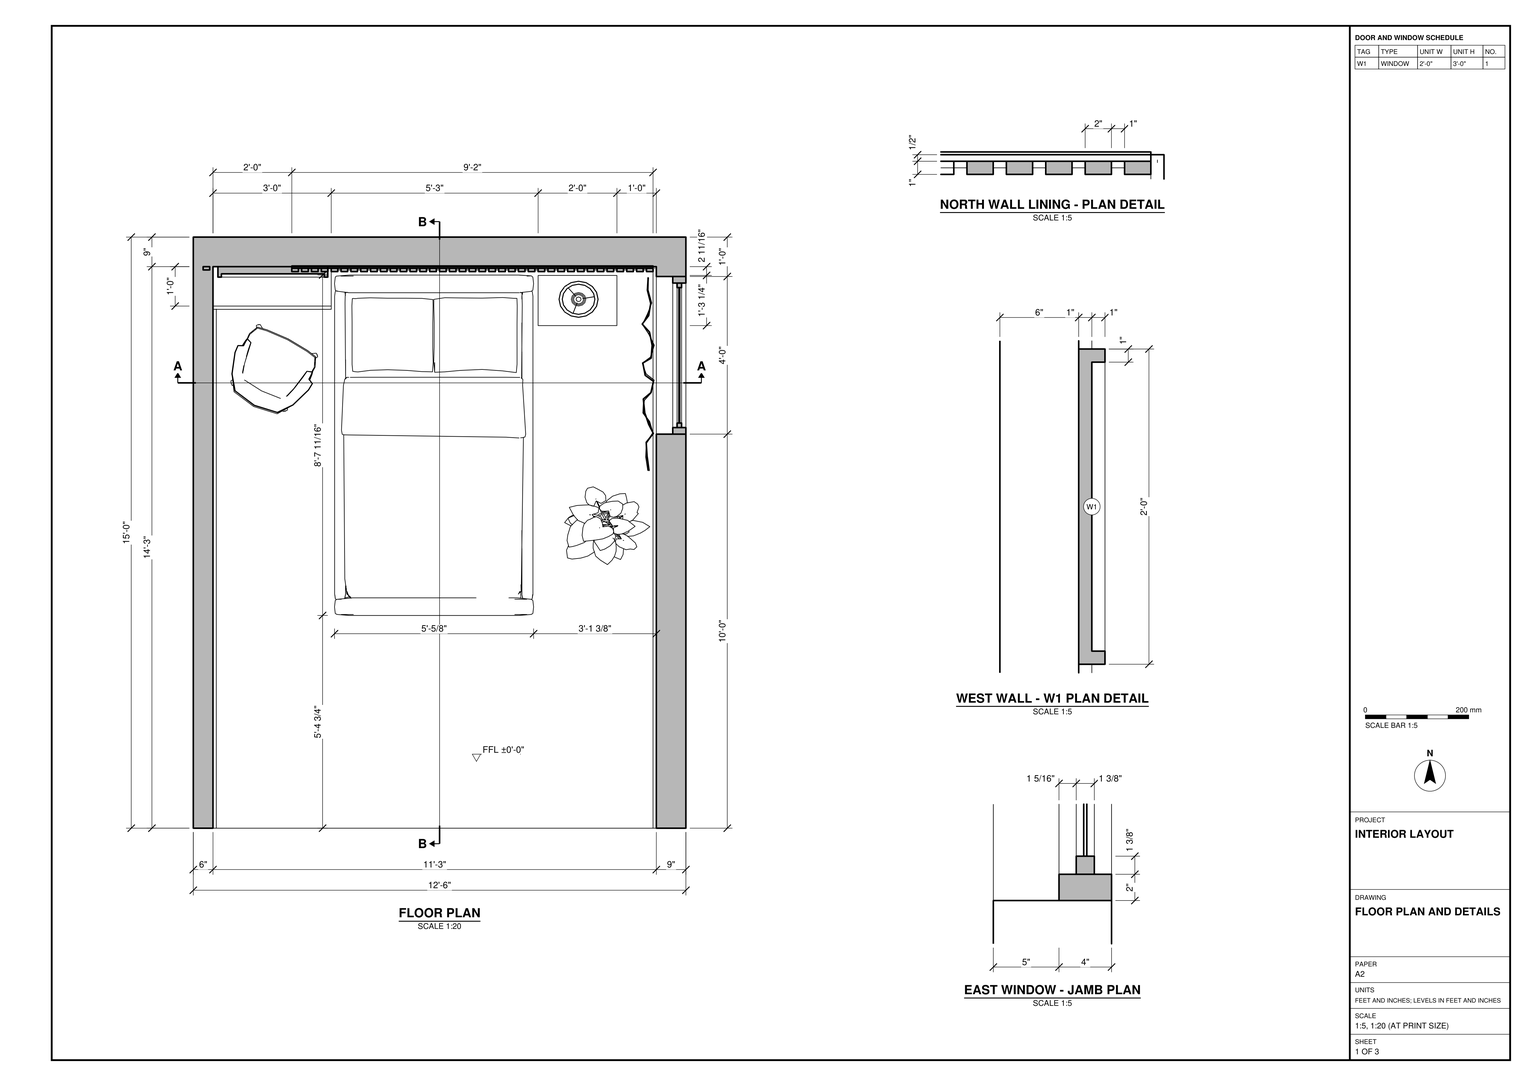
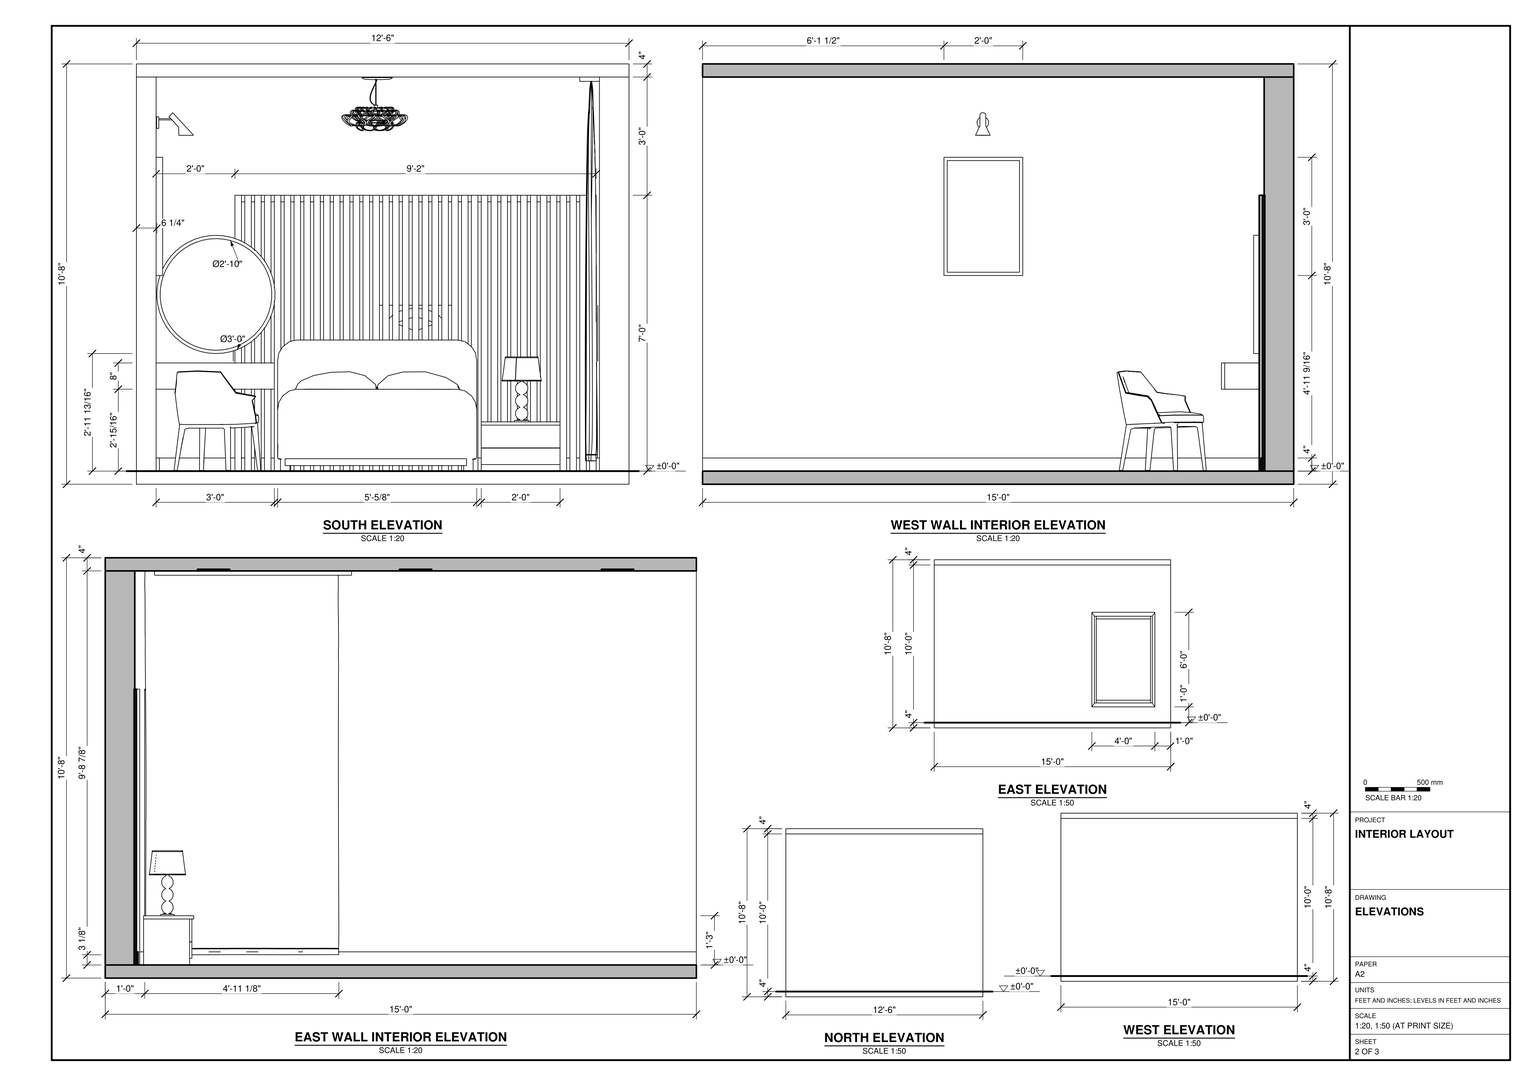
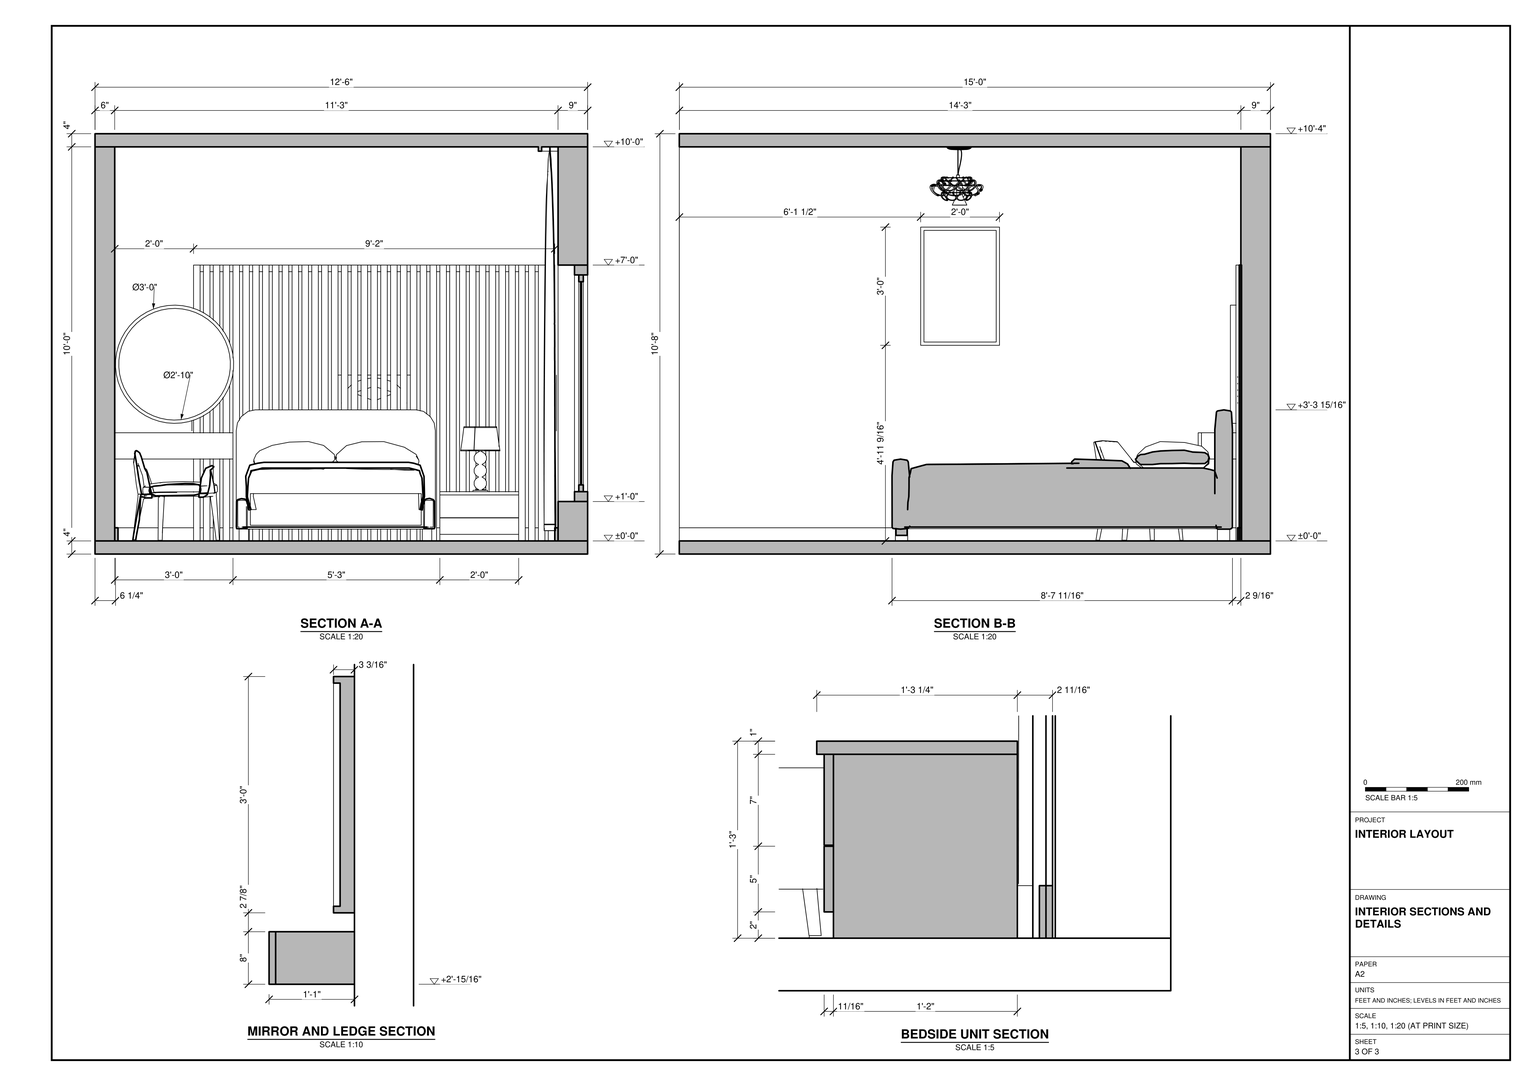
Build the bedroom in SketchUp from task_files/diagram_01.pdf. Work in feet and inches. The room shell measures 12'-6" across by 15'-0" deep and 10'-8" high overall. Set the finished floor at ±0'-0". Model the floor and ceiling slabs, each 4" thick, with a clear height of 10'-0" between them. Leave the south side open as drawn. Make the west wall 6" thick and the north and east walls 9" thick. Use the plan, elevations and jamb detail to place the east window, and include the smaller framed unit shown on the inside of the west wall.

Run the vertical slatted lining across the north wall as dimensioned. Set the bed with its head against the lining and its foot toward the open side. To the left of the bed, model the wall-mounted ledge with the round mirror above and the chair in front. To the right, model the low bedside unit using its section detail. Place the bedside lamp, curtains, plant, ceiling light and wall light where shown. Decor and loose items may be any suitable library components.

Keep the walls and slabs and each furniture or joinery piece in separate groups or components, and use components for repeated parts. Save one SketchUp model as output_files/furnished_bedroom_with_a_slatted_headboard_wall.skp.

# SketchUp Ruby script. Lengths in inches.
U = 1.inch
M = Sketchup.active_model
def pt(a) = Geom::Point3d.new(a.map { |v| v * U })
def face(e, loops, mat)
  f = e.add_face(loops[0].map { |a| pt(a) })
  loops[1..].each { |l| e.add_face(l.map { |a| pt(a) }).erase! }
  f.material = f.back_material = mat if mat
  f
end
# faces: each face lists its corners as indices into pts; further lists are holes
def faces(e, pts, list, mat = nil) = list.each { |f| face(e, (f[0].is_a?(Array) ? f : [f]).map { |l| l.map { |i| pts[i] } }, mat) }
# xy, xz, yz: faces in a plane at the given z, y or x. An outline is a flat list of corners, or four numbers for a rectangle; further outlines are holes
def ring(l) = l.size == 4 ? [[l[0], l[1]], [l[2], l[1]], [l[2], l[3]], [l[0], l[3]]] : l.each_slice(2).to_a
def flat(e, list, mat, &to3) = list.each { |f| face(e, (f[0].is_a?(Array) ? f : [f]).map { |l| ring(l).map { |u, v| to3.(u, v) } }, mat) }
def xy(e, z, list, mat = nil) = flat(e, list, mat) { |x, y| [x, y, z] }
def xz(e, y, list, mat = nil) = flat(e, list, mat) { |x, z| [x, y, z] }
def yz(e, x, list, mat = nil) = flat(e, list, mat) { |y, z| [x, y, z] }
def lines(e, pts, list) = list.each { |a, b| e.add_line(pt(pts[a]), pt(pts[b])) }
# prism: a flat outline (further loops are holes) pulled along v
def prism(e, loops, v, mat = nil)
  f = face(e, loops, mat); d = Geom::Vector3d.new(v.map { |x| x * U })
  f.pushpull(f.normal.samedirection?(d) ? d.length : -d.length)
end
def box(e, o, s, mat = nil) = prism(e, [[o, [o[0] + s[0], o[1], o[2]], [o[0] + s[0], o[1] + s[1], o[2]], [o[0], o[1] + s[1], o[2]]]], [0, 0, s[2]], mat)
def at(x, y, z, deg = 0) = Geom::Transformation.translation(pt([x, y, z])) * Geom::Transformation.rotation(ORIGIN, Z_AXIS, deg.degrees)
def axes(o, x, y, z) = Geom::Transformation.new([*x, 0, *y, 0, *z, 0, *pt(o).to_a, 1])
def part(name) = M.definitions.add(name)
# library, detail: a bought-in or finely detailed component or shape, given as its bounding box
def library(name, o, s) = part(name).tap { |d| box(d.entities, o, s) }
def detail(e, o, s) = box(e.add_group.entities, o, s)
def put(e, d, t, mat = nil) = e.add_instance(d, t).tap { |i| i.material = mat if mat }
def group(e, t, mat = nil) = e.add_group.tap { |g| g.transformation = t; g.material = mat if mat }.entities
root = M.entities
M.materials.add("0215 AP 9421 FABRIC PINK").color = [153, 66, 100]
M.materials.add("0401 AP 9656 Gulmarg Winters-N").color = [195, 225, 234]
M.materials.add("CTS Window Glass").color = [170, 210, 225]
M.materials["CTS Window Glass"].alpha = 0.45
M.materials.add("Emissive\#1").color = [255, 196, 127]
M.materials.add("[Wood Cherry Original]").color = [152, 86, 42]
c1 = part("Headboard wall slat")
box(c1.entities,[0,-4,0],[2,84,1],"[Wood Cherry Original]")
c2 = library("Light Wall 003",[-2.22,-12.37,-3.88],[4.44,12.37,6.91])
c3 = library("Chair 027",[-12.79,-10.9,0.01],[25.58,23.14,30.54])
c4 = library("Eva Bed",[-34.4,-44.85,0.04],[68.9,90.3,39.91])
c5 = library("Lamp Table 114-10",[-7.7,-7.7,0],[15.4,15.4,24.72])
c6 = library("Indoor Plant 001",[-24.46,-30.5625,0],[48.74,57.4,53.14])
c7 = library("Light",[127.07,-9.39,-4.83],[16.23,16.19,39.83])
c8 = library("Curtains 005",[1.83,-1.86,0.24],[37.77,3.72,116.83])
c9 = part("Group64\#2")
prism(c9.entities,[[[143.75,-49.45,88.01],[143.75,-51.45,86.01],[143.75,-51.45,134.01],[143.75,-49.45,132.01]]],[4,0,0])
c10 = part("Group65\#2")
prism(c10.entities,[[[143.75,-3.45,86.01],[143.75,-5.45,88.01],[143.75,-5.45,132.01],[143.75,-3.45,134.01]]],[4,0,0])
c11 = part("Group66\#2")
prism(c11.entities,[[[143.75,-49.45,132.01],[143.75,-51.45,134.01],[143.75,-3.45,134.01],[143.75,-5.45,132.01]]],[4,0,0])
c12 = part("Group67\#2")
prism(c12.entities,[[[143.75,-51.45,86.01],[143.75,-49.45,88.01],[143.75,-5.45,88.01],[143.75,-3.45,86.01]]],[4,0,0])
c13 = part("Group70\#2")
box(c13.entities,[145.0625,-49.45,88.01],[1.375,1.38,44])
c14 = part("Group71\#2")
box(c14.entities,[145.0625,-6.83,88.01],[1.375,1.38,44])
c15 = part("Group72\#2")
box(c15.entities,[145.0625,-48.07,130.64],[1.375,41.24,1.37])
c16 = part("Group73\#2")
box(c16.entities,[145.0625,-48.07,88.01],[1.375,41.24,1.38])
c17 = part("Group69\#2")
put(c17.entities,c13,at(0,0,0))
put(c17.entities,c14,at(0,0,0))
put(c17.entities,c15,at(0,0,0))
put(c17.entities,c16,at(0,0,0))
c18 = part("Group74\#2")
box(c18.entities,[145.63,-48.07,89.39],[0.24,41.24,41.25],"CTS Window Glass")
c19 = part("Group68\#2")
put(c19.entities,c17,at(0,0,0))
put(c19.entities,c18,at(0,0,0))
c20 = part("CTS_Window_Frame\#1")
put(c20.entities,c9,at(0,0,0))
put(c20.entities,c10,at(0,0,0))
put(c20.entities,c11,at(0,0,0))
put(c20.entities,c12,at(0,0,0))
put(c20.entities,c19,at(0,0,0))
c21 = library("Group\#6",[-0.5,-0.5,0],[111,1,84])
c22 = part("Recessed light pair")
xy(c22.entities,-0.5,[[5.97,1,7.27,1.16,8.47,1.66,9.51,2.44,10.32,3.47,10.82,4.68,11,5.97,10.84,7.27,10.34,8.47,9.56,9.51,8.53,10.32,7.32,10.82,6.03,11,4.73,10.84,3.53,10.34,2.49,9.56,1.68,8.53,1.18,7.32,1,6.03,1.16,4.73,1.66,3.53,2.44,2.49,3.47,1.68,4.68,1.18],[5.97,73,7.27,73.16,8.47,73.66,9.51,74.44,10.32,75.47,10.82,76.68,11,77.97,10.84,79.27,10.34,80.47,9.56,81.51,8.53,82.32,7.32,82.82,6.03,83,4.73,82.84,3.53,82.34,2.49,81.56,1.68,80.53,1.18,79.32,1,78.03,1.16,76.73,1.66,75.53,2.44,74.49,3.47,73.68,4.68,73.18]],"Emissive\#1")
xy(c22.entities,0,[[[5.96,0,7.52,0.2,8.97,0.79,10.22,1.73,11.18,2.97,11.79,4.41,12,5.96,11.8,7.52,11.21,8.97,10.27,10.22,9.03,11.18,7.59,11.79,6.04,12,4.48,11.8,3.03,11.21,1.78,10.27,0.82,9.03,0.21,7.59,0,6.04,0.2,4.48,0.79,3.03,1.73,1.78,2.97,0.82,4.41,0.21],[5.97,1,4.68,1.18,3.47,1.68,2.44,2.49,1.66,3.53,1.16,4.73,1,6.03,1.18,7.32,1.68,8.53,2.49,9.56,3.53,10.34,4.73,10.84,6.03,11,7.32,10.82,8.53,10.32,9.56,9.51,10.34,8.47,10.84,7.27,11,5.97,10.82,4.68,10.32,3.47,9.51,2.44,8.47,1.66,7.27,1.16]],[[5.96,72,7.52,72.2,8.97,72.79,10.22,73.73,11.18,74.97,11.79,76.41,12,77.96,11.8,79.52,11.21,80.97,10.27,82.22,9.03,83.18,7.59,83.79,6.04,84,4.48,83.8,3.03,83.21,1.78,82.27,0.82,81.03,0.21,79.59,0,78.04,0.2,76.48,0.79,75.03,1.73,73.78,2.97,72.82,4.41,72.21],[5.97,73,4.68,73.18,3.47,73.68,2.44,74.49,1.66,75.53,1.16,76.73,1,78.03,1.18,79.32,1.68,80.53,2.49,81.56,3.53,82.34,4.73,82.84,6.03,83,7.32,82.82,8.53,82.32,9.56,81.51,10.34,80.47,10.84,79.27,11,77.97,10.82,76.68,10.32,75.47,9.51,74.44,8.47,73.66,7.27,73.16]]])
p = [[4.68,1.18,0],[5.97,1,0],[5.97,1,-0.5],[4.68,1.18,-0.5],[7.27,1.16,0],[7.27,1.16,-0.5],
  [3.47,1.68,0],[3.47,1.68,-0.5],[8.47,1.66,0],[8.47,1.66,-0.5],[2.44,2.49,0],[2.44,2.49,-0.5],
  [9.51,2.44,0],[9.51,2.44,-0.5],[10.32,3.47,0],[10.32,3.47,-0.5],[1.66,3.53,0],[1.66,3.53,-0.5],
  [1.16,4.73,0],[1.16,4.73,-0.5],[10.82,4.68,0],[10.82,4.68,-0.5],[1,6.03,0],[1,6.03,-0.5],
  [11,5.97,0],[11,5.97,-0.5],[1.18,7.32,0],[1.18,7.32,-0.5],[10.84,7.27,0],[10.84,7.27,-0.5],
  [1.68,8.53,0],[1.68,8.53,-0.5],[10.34,8.47,0],[10.34,8.47,-0.5],[2.49,9.56,0],[2.49,9.56,-0.5],
  [9.56,9.51,0],[9.56,9.51,-0.5],[8.53,10.32,0],[8.53,10.32,-0.5],[3.53,10.34,0],[3.53,10.34,-0.5],
  [4.73,10.84,0],[4.73,10.84,-0.5],[7.32,10.82,0],[7.32,10.82,-0.5],[6.03,11,0],[6.03,11,-0.5],
  [4.68,73.18,0],[5.97,73,0],[5.97,73,-0.5],[4.68,73.18,-0.5],[7.27,73.16,0],[7.27,73.16,-0.5],
  [3.47,73.68,0],[3.47,73.68,-0.5],[8.47,73.66,0],[8.47,73.66,-0.5],[2.44,74.49,0],[2.44,74.49,-0.5],
  [9.51,74.44,0],[9.51,74.44,-0.5],[10.32,75.47,0],[10.32,75.47,-0.5],[1.66,75.53,0],[1.66,75.53,-0.5],
  [1.16,76.73,0],[1.16,76.73,-0.5],[10.82,76.68,0],[10.82,76.68,-0.5],[1,78.03,0],[1,78.03,-0.5],
  [11,77.97,0],[11,77.97,-0.5],[1.18,79.32,0],[1.18,79.32,-0.5],[10.84,79.27,0],[10.84,79.27,-0.5],
  [1.68,80.53,0],[1.68,80.53,-0.5],[10.34,80.47,0],[10.34,80.47,-0.5],[2.49,81.56,0],[2.49,81.56,-0.5],
  [9.56,81.51,0],[9.56,81.51,-0.5],[8.53,82.32,0],[8.53,82.32,-0.5],[3.53,82.34,0],[3.53,82.34,-0.5],
  [4.73,82.84,0],[4.73,82.84,-0.5],[7.32,82.82,0],[7.32,82.82,-0.5],[6.03,83,0],[6.03,83,-0.5]]
faces(c22.entities,p,[[0,1,2,3],[1,4,5,2],[6,0,3,7],[4,8,9,5],[10,6,7,11],[8,12,13,9],[12,14,15,13],[16,10,11,17],
  [18,16,17,19],[14,20,21,15],[22,18,19,23],[20,24,25,21],[26,22,23,27],[24,28,29,25],[30,26,27,31],[28,32,33,29],
  [34,30,31,35],[32,36,37,33],[36,38,39,37],[40,34,35,41],[42,40,41,43],[38,44,45,39],[46,42,43,47],[44,46,47,45],
  [48,49,50,51],[49,52,53,50],[54,48,51,55],[52,56,57,53],[58,54,55,59],[56,60,61,57],[60,62,63,61],[64,58,59,65],
  [66,64,65,67],[62,68,69,63],[70,66,67,71],[68,72,73,69],[74,70,71,75],[72,76,77,73],[78,74,75,79],[76,80,81,77],
  [82,78,79,83],[80,84,85,81],[84,86,87,85],[88,82,83,89],[90,88,89,91],[86,92,93,87],[94,90,91,95],[92,94,95,93]],"Emissive\#1")
put(root,c1,axes([3,171,4],[1,0,0],[0,0,1],[0,-1,0]))
put(root,c2,axes([6.14,85.34,106.12],[0,-1,0],[-0.91,0,0],[0,0,1]))
put(root,c3,axes([23.97,139.31,-0.01],[0.89021,-0.45554,0],[-0.45554,-0.89021,0],[0,0,1]))
put(root,c4,axes([73.27,116.26,-0.04],[0.88,0,0],[0,1.148,0],[0,0,1]))
put(root,c5,axes([117.32,161.07,15],[0.77921,0,0],[0,0.72,0],[0,0,0.8]))
put(root,c6,axes([126.09,92.88,0],[0.5325,0,0],[0,0.4125,0],[0,0,0.75]))
put(root,c7,axes([-94.8125,85.71,105.63],[1.2381,0,0],[0,1,0],[0,0,0.4107]))
put(root,c8,axes([138.53,105.99,2.86],[0,1.56501,0],[1,0,0],[0,0,1.00056]))
put(root,c20,axes([2.25,171.45,-117.02],[1,0,0],[0,1,0],[0,0,1.5]))
put(root,c1,axes([123,170.5,4],[1,0,0],[0,0,1],[0,-1,0]),"[Wood Cherry Original]")
put(root,c1,axes([108,170.5,4],[1,0,0],[0,0,1],[0,-1,0]),"[Wood Cherry Original]")
put(root,c1,axes([120,170.5,4],[1,0,0],[0,0,1],[0,-1,0]),"[Wood Cherry Original]")
put(root,c1,axes([117,170.5,4],[1,0,0],[0,0,1],[0,-1,0]),"[Wood Cherry Original]")
put(root,c1,axes([126,170.5,4],[1,0,0],[0,0,1],[0,-1,0]),"[Wood Cherry Original]")
put(root,c1,axes([135,170.5,4],[1,0,0],[0,0,1],[0,-1,0]),"[Wood Cherry Original]")
put(root,c1,axes([129,170.5,4],[1,0,0],[0,0,1],[0,-1,0]),"[Wood Cherry Original]")
put(root,c1,axes([114,170.5,4],[1,0,0],[0,0,1],[0,-1,0]),"[Wood Cherry Original]")
put(root,c1,axes([93,170.5,4],[1,0,0],[0,0,1],[0,-1,0]),"[Wood Cherry Original]")
put(root,c1,axes([111,170.5,4],[1,0,0],[0,0,1],[0,-1,0]),"[Wood Cherry Original]")
put(root,c1,axes([132,170.5,4],[1,0,0],[0,0,1],[0,-1,0]),"[Wood Cherry Original]")
put(root,c1,axes([87,170.5,4],[1,0,0],[0,0,1],[0,-1,0]),"[Wood Cherry Original]")
put(root,c1,axes([48,170.5,4],[1,0,0],[0,0,1],[0,-1,0]),"[Wood Cherry Original]")
put(root,c1,axes([75,170.5,4],[1,0,0],[0,0,1],[0,-1,0]),"[Wood Cherry Original]")
put(root,c1,axes([81,170.5,4],[1,0,0],[0,0,1],[0,-1,0]),"[Wood Cherry Original]")
put(root,c1,axes([69,170.5,4],[1,0,0],[0,0,1],[0,-1,0]),"[Wood Cherry Original]")
put(root,c1,axes([63,170.5,4],[1,0,0],[0,0,1],[0,-1,0]),"[Wood Cherry Original]")
put(root,c1,axes([90,170.5,4],[1,0,0],[0,0,1],[0,-1,0]),"[Wood Cherry Original]")
put(root,c1,axes([57,170.5,4],[1,0,0],[0,0,1],[0,-1,0]),"[Wood Cherry Original]")
put(root,c1,axes([60,170.5,4],[1,0,0],[0,0,1],[0,-1,0]),"[Wood Cherry Original]")
put(root,c1,axes([84,170.5,4],[1,0,0],[0,0,1],[0,-1,0]),"[Wood Cherry Original]")
put(root,c1,axes([51,170.5,4],[1,0,0],[0,0,1],[0,-1,0]),"[Wood Cherry Original]")
put(root,c1,axes([78,170.5,4],[1,0,0],[0,0,1],[0,-1,0]),"[Wood Cherry Original]")
put(root,c1,axes([66,170.5,4],[1,0,0],[0,0,1],[0,-1,0]),"[Wood Cherry Original]")
put(root,c1,axes([72,170.5,4],[1,0,0],[0,0,1],[0,-1,0]),"[Wood Cherry Original]")
put(root,c1,axes([54,170.5,4],[1,0,0],[0,0,1],[0,-1,0]),"[Wood Cherry Original]")
put(root,c1,axes([39,170.5,4],[1,0,0],[0,0,1],[0,-1,0]),"[Wood Cherry Original]")
put(root,c1,axes([36,170.5,4],[1,0,0],[0,0,1],[0,-1,0]),"[Wood Cherry Original]")
put(root,c1,axes([30,170.5,4],[1,0,0],[0,0,1],[0,-1,0]),"[Wood Cherry Original]")
put(root,c1,axes([33,170.5,4],[1,0,0],[0,0,1],[0,-1,0]),"[Wood Cherry Original]")
put(root,c1,axes([42,170.5,4],[1,0,0],[0,0,1],[0,-1,0]),"[Wood Cherry Original]")
put(root,c1,axes([138,170.5,4],[1,0,0],[0,0,1],[0,-1,0]),"[Wood Cherry Original]")
put(root,c1,axes([45,170.5,4],[1,0,0],[0,0,1],[0,-1,0]),"[Wood Cherry Original]")
put(root,c1,axes([99,170.5,4],[1,0,0],[0,0,1],[0,-1,0]),"[Wood Cherry Original]")
put(root,c1,axes([96,170.5,4],[1,0,0],[0,0,1],[0,-1,0]),"[Wood Cherry Original]")
put(root,c1,axes([102,170.5,4],[1,0,0],[0,0,1],[0,-1,0]),"[Wood Cherry Original]")
put(root,c1,axes([105,170.5,4],[1,0,0],[0,0,1],[0,-1,0]),"[Wood Cherry Original]")
g1 = group(root,at(6,180,0,-90))
prism(g1,[[[0,-6,0],[0,0,0],[0,144,0],[0,144,-4],[0,-6,-4]]],[180,0,0])
g2 = group(root,at(6,0,0))
prism(g2,[[[135,171,0],[135,0,0],[134,0,0],[134,170,0],[1,170,0],[1,0,0],[0,0,0],[0,171,0]]],[0,0,4])
g3 = group(root,at(0,0,0))
xy(g3,0,[[0,0,0,180,150,180,150,0,141,0,141,171,6,171,6,0]])
xy(g3,12,[[141,120,150,168]])
xy(g3,84,[[141,120,150,168]])
xy(g3,120,[[0,0,6,0,6,171,141,171,141,0,150,0,150,180,0,180]])
xz(g3,0,[[0,0,6,120],[141,0,150,120]])
xz(g3,120,[[141,12,150,84]])
xz(g3,168,[[141,12,150,84]])
xz(g3,171,[[6,0,141,120]],"0401 AP 9656 Gulmarg Winters-N")
xz(g3,180,[[0,0,150,120]])
yz(g3,0,[[0,0,180,120]])
yz(g3,6,[[0,0,171,120]],"0401 AP 9656 Gulmarg Winters-N")
yz(g3,141,[[[0,0,171,120],[120,12,168,84]]],"0401 AP 9656 Gulmarg Winters-N")
yz(g3,150,[[[0,0,180,120],[120,12,168,84]]])
g4 = group(g3,at(6,73.5,59.5625))
xy(g4,0,[[0,0,2,24]])
xy(g4,1,[[1,1,2,23]])
xy(g4,35,[[1,1,2,23]])
xy(g4,36,[[0,0,2,24]])
xz(g4,0,[[0,0,2,36]])
xz(g4,1,[[1,1,2,35]])
xz(g4,23,[[1,1,2,35]])
xz(g4,24,[[0,0,2,36]])
yz(g4,0,[[0,0,24,36]])
yz(g4,1,[[1,1,23,35]])
yz(g4,2,[[[0,0,24,36],[1,1,23,35]]])
put(root,c21,at(30,170.5,0))
g5 = group(root,at(6.25,167.8125,35.8),"0215 AP 9421 FABRIC PINK")
xz(g5,0,[[[17.79,0,20.05,0.12,22.27,0.52,24.43,1.2,26.49,2.14,28.41,3.33,30.16,4.75,31.73,6.38,33.07,8.2,34.18,10.17,35.04,12.26,35.62,14.45,35.93,16.69,35.95,18.95,35.69,21.19,35.15,23.39,34.34,25.5,33.27,27.49,31.96,29.33,30.43,30.99,28.7,32.45,26.81,33.68,24.77,34.67,22.63,35.39,20.41,35.83,18.16,36,15.9,35.88,13.68,35.48,11.52,34.8,9.47,33.86,7.54,32.67,5.79,31.25,4.22,29.61,2.875,27.8,1.77,25.83,0.91,23.74,0.33,21.55,0.02,19.3125,0,17.05,0.26,14.81,0.8,12.61,1.61,10.5,2.68,8.51,3.99,6.67,5.52,5,7.25,3.55,9.14,2.31,11.18,1.33,13.32,0.61,15.54,0.16],[17.8,1,15.67,1.16,13.58,1.58,11.56,2.26,9.63,3.1875,7.84,4.35,6.21,5.73,4.77,7.3,3.53,9.04,2.52,10.92,1.75,12.91,1.24,14.98,1,17.11,1.02,19.24,1.31,21.36,1.86,23.42,2.67,25.39,3.72,27.25,4.99,28.97,6.47,30.51,8.125,31.85,9.9375,32.98,11.88,33.87,13.92,34.51,16.02,34.89,18.15,35,20.28,34.84,22.37,34.42,24.39,33.74,26.32,32.8125,28.11,31.65,29.74,30.27,31.18,28.7,32.42,26.96,33.43,25.08,34.2,23.09,34.71,21.01,34.95,18.89,34.93,16.76,34.64,14.64,34.09,12.58,33.28,10.6,32.23,8.74,30.96,7.03,29.49,5.49,27.83,4.14,26.01,3.02,24.07,2.13,22.03,1.49,19.93,1.11]]])
xz(g5,1,[[17.8,1,19.93,1.11,22.03,1.49,24.07,2.13,26.01,3.02,27.83,4.14,29.49,5.49,30.96,7.03,32.23,8.74,33.28,10.6,34.09,12.58,34.64,14.64,34.93,16.76,34.95,18.89,34.71,21.01,34.2,23.09,33.43,25.08,32.42,26.96,31.18,28.7,29.74,30.27,28.11,31.65,26.32,32.8125,24.39,33.74,22.37,34.42,20.28,34.84,18.15,35,16.02,34.89,13.92,34.51,11.88,33.87,9.9375,32.98,8.125,31.85,6.47,30.51,4.99,28.97,3.72,27.25,2.67,25.39,1.86,23.42,1.31,21.36,1.02,19.24,1,17.11,1.24,14.98,1.75,12.91,2.52,10.92,3.53,9.04,4.77,7.3,6.21,5.73,7.84,4.35,9.63,3.1875,11.56,2.26,13.58,1.58,15.67,1.16]])
xz(g5,3.1875,[[17.79,0,15.54,0.16,13.32,0.61,11.18,1.33,9.14,2.31,7.25,3.55,5.52,5,3.99,6.67,2.68,8.51,1.61,10.5,0.8,12.61,0.26,14.81,0,17.05,0.02,19.3125,0.33,21.55,0.91,23.74,1.77,25.83,2.875,27.8,4.22,29.61,5.79,31.25,7.54,32.67,9.47,33.86,11.52,34.8,13.68,35.48,15.9,35.88,18.16,36,20.41,35.83,22.63,35.39,24.77,34.67,26.81,33.68,28.7,32.45,30.43,30.99,31.96,29.33,33.27,27.49,34.34,25.5,35.15,23.39,35.69,21.19,35.95,18.95,35.93,16.69,35.62,14.45,35.04,12.26,34.18,10.17,33.07,8.2,31.73,6.38,30.16,4.75,28.41,3.33,26.49,2.14,24.43,1.2,22.27,0.52,20.05,0.12]])
p = [[15.54,3.1875,0.16],[17.79,3.1875,0],[17.79,0,0],[15.54,0,0.16],[20.05,3.1875,0.12],[20.05,0,0.12],
  [22.27,3.1875,0.52],[22.27,0,0.52],[13.32,3.1875,0.61],[13.32,0,0.61],[24.43,3.1875,1.2],[24.43,0,1.2],
  [11.18,3.1875,1.33],[11.18,0,1.33],[15.67,0,1.16],[17.8,0,1],[17.8,1,1],[15.67,1,1.16],
  [19.93,0,1.11],[19.93,1,1.11],[22.03,0,1.49],[22.03,1,1.49],[13.58,0,1.58],[13.58,1,1.58],
  [26.49,3.1875,2.14],[26.49,0,2.14],[9.14,3.1875,2.31],[9.14,0,2.31],[24.07,0,2.13],[24.07,1,2.13],
  [11.56,0,2.26],[11.56,1,2.26],[26.01,0,3.02],[26.01,1,3.02],[28.41,3.1875,3.33],[28.41,0,3.33],
  [7.25,3.1875,3.55],[7.25,0,3.55],[9.63,0,3.1875],[9.63,1,3.1875],[27.83,0,4.14],[27.83,1,4.14],
  [7.84,0,4.35],[7.84,1,4.35],[30.16,3.1875,4.75],[30.16,0,4.75],[5.52,3.1875,5],[5.52,0,5],
  [29.49,0,5.49],[29.49,1,5.49],[6.21,0,5.73],[6.21,1,5.73],[31.73,3.1875,6.38],[31.73,0,6.38],
  [3.99,3.1875,6.67],[3.99,0,6.67],[30.96,0,7.03],[30.96,1,7.03],[4.77,0,7.3],[4.77,1,7.3],
  [33.07,3.1875,8.2],[33.07,0,8.2],[2.68,3.1875,8.51],[2.68,0,8.51],[32.23,0,8.74],[32.23,1,8.74],
  [3.53,0,9.04],[3.53,1,9.04],[34.18,3.1875,10.17],[34.18,0,10.17],[1.61,3.1875,10.5],[1.61,0,10.5],
  [33.28,0,10.6],[33.28,1,10.6],[2.52,0,10.92],[2.52,1,10.92],[35.04,3.1875,12.26],[35.04,0,12.26],
  [0.8,3.1875,12.61],[0.8,0,12.61],[34.09,0,12.58],[34.09,1,12.58],[1.75,0,12.91],[1.75,1,12.91],
  [35.62,3.1875,14.45],[35.62,0,14.45],[0.26,3.1875,14.81],[0.26,0,14.81],[34.64,0,14.64],[34.64,1,14.64],
  [1.24,0,14.98],[1.24,1,14.98],[35.93,3.1875,16.69],[35.93,0,16.69],[34.93,0,16.76],[34.93,1,16.76],
  [0,3.1875,17.05],[0,0,17.05],[1,0,17.11],[1,1,17.11],[35.95,3.1875,18.95],[35.95,0,18.95],
  [34.95,0,18.89],[34.95,1,18.89],[0.02,3.1875,19.3125],[0.02,0,19.3125],[1.02,0,19.24],[1.02,1,19.24],
  [34.71,0,21.01],[34.71,1,21.01],[35.69,3.1875,21.19],[35.69,0,21.19],[1.31,0,21.36],[1.31,1,21.36],
  [0.33,3.1875,21.55],[0.33,0,21.55],[34.2,0,23.09],[34.2,1,23.09],[35.15,3.1875,23.39],[35.15,0,23.39],
  [1.86,0,23.42],[1.86,1,23.42],[0.91,3.1875,23.74],[0.91,0,23.74],[33.43,0,25.08],[33.43,1,25.08],
  [2.67,0,25.39],[2.67,1,25.39],[34.34,3.1875,25.5],[34.34,0,25.5],[1.77,3.1875,25.83],[1.77,0,25.83],
  [32.42,0,26.96],[32.42,1,26.96],[3.72,0,27.25],[3.72,1,27.25],[33.27,3.1875,27.49],[33.27,0,27.49],
  [2.875,3.1875,27.8],[2.875,0,27.8],[31.18,0,28.7],[31.18,1,28.7],[4.99,0,28.97],[4.99,1,28.97],
  [31.96,3.1875,29.33],[31.96,0,29.33],[4.22,3.1875,29.61],[4.22,0,29.61],[29.74,0,30.27],[29.74,1,30.27],
  [6.47,0,30.51],[6.47,1,30.51],[30.43,3.1875,30.99],[30.43,0,30.99],[5.79,3.1875,31.25],[5.79,0,31.25],
  [28.11,0,31.65],[28.11,1,31.65],[8.125,0,31.85],[8.125,1,31.85],[28.7,3.1875,32.45],[28.7,0,32.45],
  [7.54,3.1875,32.67],[7.54,0,32.67],[26.32,0,32.8125],[26.32,1,32.8125],[9.9375,0,32.98],[9.9375,1,32.98],
  [26.81,3.1875,33.68],[26.81,0,33.68],[9.47,3.1875,33.86],[9.47,0,33.86],[24.39,0,33.74],[24.39,1,33.74],
  [11.88,0,33.87],[11.88,1,33.87],[22.37,0,34.42],[22.37,1,34.42],[24.77,3.1875,34.67],[24.77,0,34.67],
  [11.52,3.1875,34.8],[11.52,0,34.8],[13.92,0,34.51],[13.92,1,34.51],[20.28,0,34.84],[20.28,1,34.84],
  [16.02,0,34.89],[16.02,1,34.89],[22.63,3.1875,35.39],[22.63,0,35.39],[13.68,3.1875,35.48],[13.68,0,35.48],
  [18.15,0,35],[18.15,1,35],[20.41,3.1875,35.83],[20.41,0,35.83],[15.9,3.1875,35.88],[15.9,0,35.88],
  [18.16,3.1875,36],[18.16,0,36]]
faces(g5,p,[[0,1,2,3],[1,4,5,2],[4,6,7,5],[8,0,3,9],[6,10,11,7],[12,8,9,13],[14,15,16,17],[15,18,19,16],
  [18,20,21,19],[22,14,17,23],[10,24,25,11],[26,12,13,27],[20,28,29,21],[30,22,23,31],[28,32,33,29],[24,34,35,25],
  [36,26,27,37],[38,30,31,39],[32,40,41,33],[42,38,39,43],[34,44,45,35],[46,36,37,47],[40,48,49,41],[50,42,43,51],
  [44,52,53,45],[54,46,47,55],[48,56,57,49],[58,50,51,59],[52,60,61,53],[62,54,55,63],[56,64,65,57],[66,58,59,67],
  [60,68,69,61],[70,62,63,71],[64,72,73,65],[74,66,67,75],[68,76,77,69],[78,70,71,79],[72,80,81,73],[82,74,75,83],
  [76,84,85,77],[86,78,79,87],[80,88,89,81],[90,82,83,91],[84,92,93,85],[88,94,95,89],[96,86,87,97],[98,90,91,99],
  [92,100,101,93],[94,102,103,95],[104,96,97,105],[106,98,99,107],[102,108,109,103],[100,110,111,101],[112,106,107,113],[114,104,105,115],
  [108,116,117,109],[110,118,119,111],[120,112,113,121],[122,114,115,123],[116,124,125,117],[126,120,121,127],[118,128,129,119],[130,122,123,131],
  [124,132,133,125],[134,126,127,135],[128,136,137,129],[138,130,131,139],[132,140,141,133],[142,134,135,143],[136,144,145,137],[146,138,139,147],
  [140,148,149,141],[150,142,143,151],[144,152,153,145],[154,146,147,155],[148,156,157,149],[158,150,151,159],[152,160,161,153],[162,154,155,163],
  [156,164,165,157],[166,158,159,167],[160,168,169,161],[170,162,163,171],[164,172,173,165],[174,166,167,175],[172,176,177,173],[168,178,179,169],
  [180,170,171,181],[182,174,175,183],[176,184,185,177],[186,182,183,187],[178,188,189,179],[190,180,181,191],[184,192,193,185],[192,186,187,193],
  [188,194,195,189],[196,190,191,197],[194,198,199,195],[198,196,197,199]])
g6 = group(root,at(6,171,24.9375))
box(g6,[0,-12,0],[36,12,8])
g7 = group(root,at(6,159,24.9375))
box(g7,[0,-1,0],[36,1,8])
g8 = group(root,at(105,154.32,0))
prism(g8,[[[0,14,0],[0,0,0],[0,0,2],[0,0,7],[0,0,7.08],[0,0,14],[0,14,14]]],[24,0,0])
g9 = group(root,at(105,154.32,7.08))
box(g9,[0,-0.71,0],[24,0.71,6.92])
g10 = group(root,at(105,154.32,2))
box(g10,[0,-0.71,0],[24,0.71,5])
g11 = group(root,at(105,153.61,14))
box(g11,[0,-0.5625,0],[24,15.27,1])
g12 = group(root,at(6,180,124,-90))
xy(g12,-5.3125,[[15,129,15,135,16,135,16,130,74,130,74,135,75,135,75,129]])
xy(g12,-4,[[[0,-6,180,144],[15,129,75,129,75,135,74,135,74,130,16,130,16,135,15,135]]])
xy(g12,0,[[0,-6,180,144]])
xz(g12,-6,[[0,-4,180,0]])
xz(g12,129,[[15,-5.3125,75,-4]])
xz(g12,130,[[16,-5.3125,74,-4]])
xz(g12,135,[[15,-5.3125,16,-4],[74,-5.3125,75,-4]])
xz(g12,144,[[0,-4,180,0]])
yz(g12,0,[[-6,-4,144,0]])
yz(g12,15,[[129,-5.3125,135,-4]])
yz(g12,16,[[130,-5.3125,135,-4]])
yz(g12,74,[[130,-5.3125,135,-4]])
yz(g12,75,[[129,-5.3125,135,-4]])
yz(g12,180,[[-6,-4,144,0]])
put(g12,c22,axes([39,21,-4],[-1,0,0],[0,1,0],[0,0,-1]))
put(g12,c22,axes([100.5,21,-4],[-1,0,0],[0,1,0],[0,0,-1]))
put(g12,c22,axes([162,21,-4],[-1,0,0],[0,1,0],[0,0,-1]))
g13 = group(root,at(30,170.5,0))
box(g13,[0,0,0],[110,0.71,84])
